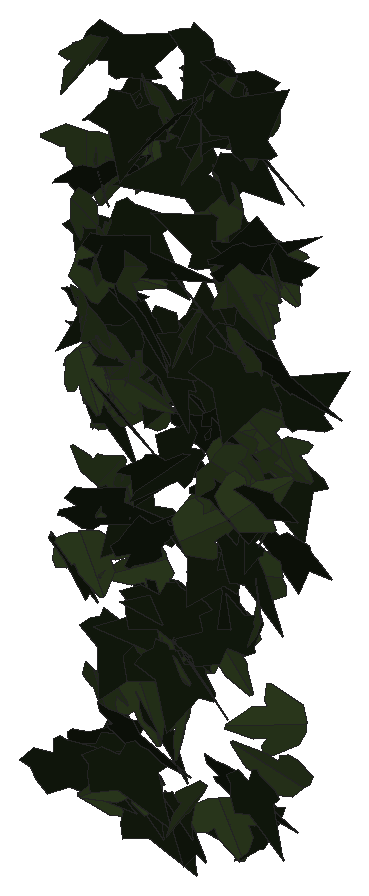
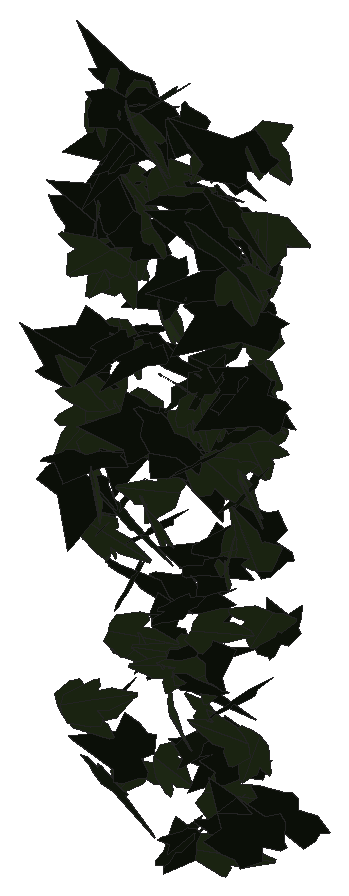
# SketchUp Ruby script. Lengths in inches.
U = 1.inch
M = Sketchup.active_model
def pt(a) = Geom::Point3d.new(a.map { |v| v * U })
def face(e, loops, mat)
  f = e.add_face(loops[0].map { |a| pt(a) })
  loops[1..].each { |l| e.add_face(l.map { |a| pt(a) }).erase! }
  f.material = f.back_material = mat if mat
  f
end
# faces: each face lists its corners as indices into pts; further lists are holes
def faces(e, pts, list, mat = nil) = list.each { |f| face(e, (f[0].is_a?(Array) ? f : [f]).map { |l| l.map { |i| pts[i] } }, mat) }
# xy, xz, yz: faces in a plane at the given z, y or x. An outline is a flat list of corners, or four numbers for a rectangle; further outlines are holes
def ring(l) = l.size == 4 ? [[l[0], l[1]], [l[2], l[1]], [l[2], l[3]], [l[0], l[3]]] : l.each_slice(2).to_a
def flat(e, list, mat, &to3) = list.each { |f| face(e, (f[0].is_a?(Array) ? f : [f]).map { |l| ring(l).map { |u, v| to3.(u, v) } }, mat) }
def xy(e, z, list, mat = nil) = flat(e, list, mat) { |x, y| [x, y, z] }
def xz(e, y, list, mat = nil) = flat(e, list, mat) { |x, z| [x, y, z] }
def yz(e, x, list, mat = nil) = flat(e, list, mat) { |y, z| [x, y, z] }
def lines(e, pts, list) = list.each { |a, b| e.add_line(pt(pts[a]), pt(pts[b])) }
# prism: a flat outline (further loops are holes) pulled along v
def prism(e, loops, v, mat = nil)
  f = face(e, loops, mat); d = Geom::Vector3d.new(v.map { |x| x * U })
  f.pushpull(f.normal.samedirection?(d) ? d.length : -d.length)
end
def box(e, o, s, mat = nil) = prism(e, [[o, [o[0] + s[0], o[1], o[2]], [o[0] + s[0], o[1] + s[1], o[2]], [o[0], o[1] + s[1], o[2]]]], [0, 0, s[2]], mat)
def at(x, y, z, deg = 0) = Geom::Transformation.translation(pt([x, y, z])) * Geom::Transformation.rotation(ORIGIN, Z_AXIS, deg.degrees)
def axes(o, x, y, z) = Geom::Transformation.new([*x, 0, *y, 0, *z, 0, *pt(o).to_a, 1])
def part(name) = M.definitions.add(name)
# library, detail: a bought-in or finely detailed component or shape, given as its bounding box
def library(name, o, s) = part(name).tap { |d| box(d.entities, o, s) }
def detail(e, o, s) = box(e.add_group.entities, o, s)
def put(e, d, t, mat = nil) = e.add_instance(d, t).tap { |i| i.material = mat if mat }
def group(e, t, mat = nil) = e.add_group.tap { |g| g.transformation = t; g.material = mat if mat }.entities
root = M.entities
M.materials.add("1026 AP 7946 SUNNY SIDE UP").color = [254, 231, 186]
M.materials.add("efeu1").color = [18, 25, 13]
M.materials.add("efeu2").color = [43, 57, 29]
c1 = part("ivyleaf_10")
p = [[0,0.5,-0.03],[-0.0625,2.02,-0.43],[-0.19,2.01,-0.46],[-0.54,1.05,-0.29],[-0.52,0.625,-0.18],[-0.83,0.76,-0.28],
  [-1.16,0.64,-0.33],[-1.15,0.33,-0.24],[-0.77,-0.39,0.02],[-0.3,-0.51,0.16],[0.04,-0.48,0.23],[-0.02,2.01,-0.4375],
  [-0.06,2.01,-0.43],[0.04,-0.49,0.23],[0.67,-0.49,0.14],[1.38,0.36,-0.2],[1.375,0.51,-0.24],[0.81,0.65,-0.19],
  [0.62,0.59,-0.15],[0.6,1.09,-0.28],[0.5,1.23,-0.31]]
faces(c1.entities,p,[[0,1,2,3,4,5,6,7,8,9,10],[11,12,0,13,14,15,16,17,18,19,20]],"efeu2")
c2 = part("ivyleaf_9")
p = [[1.54,2.16,1.25],[1.36,2.04,1.19],[-0.21,0.99,0.68],[-0.71,1.11,0.82],[-0.85,0.86,0.67],[-0.8,0.17,0.21],
  [-0.9,-0.01,0.1],[-0.67,-0.16,-0.02],[-0.08,-0.08,-0.05],[-0.03,-0.6,-0.4],[0.65,-0.88,-0.66],[0.83,-0.6,-0.49],
  [1.29,-0.42,-0.43],[1.8125,-0.07,-0.26],[1.21,0.44,0.15]]
faces(c2.entities,p,[[0,1,2,3,4,5,6,7,8,9,10,11,12,13,14]],"efeu1")
put(root,c1,axes([125.12,211.6,276.24],[-0.30971,0.08438,0.28266],[0.40804,-0.08857,0.21984],[0.1913,0.32553,-0.01128]),"1026 AP 7946 SUNNY SIDE UP")
put(root,c2,axes([126.02,211.5,273.74],[0.08468,0.26535,-0.18565],[-0.0411,-0.18002,-0.27985],[-0.50402,0.05926,-0.00837]),"1026 AP 7946 SUNNY SIDE UP")
put(root,c2,axes([126.16,211.55,278.82],[-0.20277,0.23701,-0.16333],[0.09037,-0.15033,-0.2782],[-0.44036,-0.13998,0.01811]),"1026 AP 7946 SUNNY SIDE UP")
put(root,c1,axes([127,211.62,276.72],[-0.33741,0.11008,-0.27658],[0.31923,-0.18267,-0.24483],[-0.32724,-0.2917,0.04633]),"1026 AP 7946 SUNNY SIDE UP")
put(root,c2,axes([127.09,211.51,278.92],[-0.22211,0.14991,0.2901],[0.32473,-0.19053,0.21075],[0.38078,0.24994,-0.01051]),"1026 AP 7946 SUNNY SIDE UP")
put(root,c2,axes([125.28,211.53,269.14],[-0.03055,-0.2161,-0.22105],[0.11388,0.20432,-0.21881],[0.46372,-0.06441,0.03917]),"1026 AP 7946 SUNNY SIDE UP")
put(root,c1,axes([126.95,211.41,274.0625],[-0.13765,-0.21772,-0.24],[0.20403,0.19497,-0.23807],[0.45645,-0.15281,0.03404]),"1026 AP 7946 SUNNY SIDE UP")
put(root,c2,axes([124.92,211.61,274.3],[0.3457,-0.17847,0.06715],[0.05909,-0.05845,-0.29125],[0.29342,0.22204,-0.02047]),"1026 AP 7946 SUNNY SIDE UP")
put(root,c1,axes([126.33,211.6875,275.83],[0.15419,-0.27095,0.12188],[0.04264,-0.1175,-0.29722],[0.46391,0.10086,-0.01319]),"1026 AP 7946 SUNNY SIDE UP")
put(root,c2,axes([127.31,211.62,269.43],[0.16228,-0.2843,-0.07382],[-0.06451,0.05949,-0.3107],[0.45586,0.10963,-0.01769]),"1026 AP 7946 SUNNY SIDE UP")
put(root,c2,axes([127.18,211.46,273.73],[0.42834,0.15969,-0.14948],[-0.17686,-0.09604,-0.32496],[-0.29066,0.29378,-0.02257]),"1026 AP 7946 SUNNY SIDE UP")
put(root,c2,axes([125.08,211.39,276.48],[0.39253,0.08741,0.26918],[0.40942,0.0384,-0.2698],[-0.13938,0.35897,-0.03444]),"1026 AP 7946 SUNNY SIDE UP")
put(root,c1,axes([125.26,211.59,274.625],[0.03815,-0.00602,0.29977],[0.45738,0.01135,-0.02468],[-0.01701,0.29181,0.00886]),"1026 AP 7946 SUNNY SIDE UP")
put(root,c2,axes([124.73,211.4,272.69],[0.34005,0.10747,0.23171],[0.34174,0.06289,-0.24654],[-0.19017,0.30517,-0.02871]),"1026 AP 7946 SUNNY SIDE UP")
put(root,c2,axes([127.09,211.78,275.27],[-0.23418,-0.2826,0.02912],[-0.00061,-0.03352,-0.32891],[0.44683,-0.14815,0.01481]),"1026 AP 7946 SUNNY SIDE UP")
put(root,c2,axes([124.88,211.5,277.64],[0.11895,0.28671,-0.08881],[-0.0333,-0.08525,-0.30597],[-0.47032,0.07855,-0.0008]),"1026 AP 7946 SUNNY SIDE UP")
put(root,c1,axes([125.05,211.35,276.43],[0.10038,-0.0414,0.37634],[-0.32327,0.30365,0.07419],[-0.47969,-0.2133,0.02875]),"1026 AP 7946 SUNNY SIDE UP")
put(root,c2,axes([124.24,211.83,271.49],[-0.00484,-0.17117,0.26038],[0.10676,-0.24779,-0.17282],[0.46926,0.05461,0.042]),"1026 AP 7946 SUNNY SIDE UP")
put(root,c1,axes([126.29,211.79,268.85],[0.06161,-0.21932,0.21022],[0.03119,-0.2047,-0.23038],[0.47135,0.04221,-0.01223]),"1026 AP 7946 SUNNY SIDE UP")
put(root,c2,axes([126.1875,211.66,276.29],[0.39564,-0.19646,0.02072],[0.00176,-0.03295,-0.32803],[0.3107,0.25035,-0.02452]),"1026 AP 7946 SUNNY SIDE UP")
put(root,c2,axes([126.23,211.7,273.91],[-0.46209,0.13322,-0.12073],[0.14856,-0.07614,-0.33155],[-0.23707,-0.30737,0.02755]),"1026 AP 7946 SUNNY SIDE UP")
put(root,c2,axes([125.85,211.63,271.64],[-0.14687,-0.12827,-0.27634],[0.31991,0.17642,-0.1593],[0.33952,-0.22173,0.03056]),"1026 AP 7946 SUNNY SIDE UP")
put(root,c2,axes([126.53,211.87,272.42],[-0.1496,-0.25042,0.15774],[-0.05748,-0.1511,-0.27631],[0.45912,-0.10051,0.01681]),"1026 AP 7946 SUNNY SIDE UP")
put(root,c2,axes([125.33,211.76,278.52],[-0.37869,-0.07665,-0.18426],[0.29452,-0.01666,-0.25318],[0.08059,-0.29927,0.05941]),"1026 AP 7946 SUNNY SIDE UP")
put(root,c1,axes([126.55,211.49,278.5625],[0.06983,-0.26487,-0.2432],[-0.03165,0.23414,-0.27492],[0.55542,0.04664,0.01491]),"1026 AP 7946 SUNNY SIDE UP")
put(root,c1,axes([127.29,211.43,273.54],[0.19729,0.10733,-0.30542],[0.30849,0.22405,0.17006],[0.38926,-0.23195,0.02003]),"1026 AP 7946 SUNNY SIDE UP")
put(root,c1,axes([125.33,211.84,268.78],[0.15458,0.07911,-0.33089],[-0.33001,-0.24469,-0.12951],[-0.40293,0.23075,-0.02087]),"1026 AP 7946 SUNNY SIDE UP")
put(root,c2,axes([124.18,211.59,268.77],[0.0055,-0.05249,-0.31572],[0.32346,0.22983,-0.03683],[0.366,-0.20232,0.03729]),"1026 AP 7946 SUNNY SIDE UP")
put(root,c1,axes([124.83,211.64,275.13],[-0.43077,0.1254,-0.02626],[0.02055,-0.03418,-0.30947],[-0.20038,-0.27308,0.02472]),"1026 AP 7946 SUNNY SIDE UP")
put(root,c1,axes([124.71,211.6,275.43],[-0.36428,0.14915,0.1485],[-0.21635,0.04953,-0.28197],[-0.24283,-0.26787,0.02844]),"1026 AP 7946 SUNNY SIDE UP")
put(root,c2,axes([126.23,211.65,270.92],[0.39463,-0.13734,-0.10286],[-0.15431,0.02637,-0.29365],[0.21699,0.26852,-0.02177]),"1026 AP 7946 SUNNY SIDE UP")
put(root,c1,axes([124.56,211.84,279.16],[-0.00909,-0.30607,0.16579],[-0.01714,-0.16245,-0.31624],[0.54475,-0.01022,-0.00718]),"1026 AP 7946 SUNNY SIDE UP")
put(root,c2,axes([126.375,211.85,277.93],[-0.39497,-0.05239,0.1896],[-0.2686,-0.07657,-0.26265],[0.13661,-0.30202,0.03176]),"1026 AP 7946 SUNNY SIDE UP")
put(root,c1,axes([126.47,211.47,272.87],[0.10422,0.06933,-0.33181],[0.3061,0.2573,0.09971],[0.41868,-0.20537,0.0097]),"1026 AP 7946 SUNNY SIDE UP")
put(root,c2,axes([127.05,211.5,277],[0.18894,0.28554,-0.15961],[0.04138,0.15781,0.31826],[0.51037,-0.1185,0.03329]),"1026 AP 7946 SUNNY SIDE UP")
put(root,c1,axes([127.53,211.49,272.04],[0.01747,-0.10018,-0.32543],[-0.11646,0.30674,-0.10129],[0.50703,0.07391,-0.01205]),"1026 AP 7946 SUNNY SIDE UP")
put(root,c2,axes([125.98,211.9,270.5625],[-0.15623,-0.28157,0.05652],[-0.01499,-0.05648,-0.30777],[0.4513,-0.09935,0.00934]),"1026 AP 7946 SUNNY SIDE UP")
put(root,c2,axes([126.95,211.57,271.37],[-0.5334,0.05893,-0.07586],[-0.10529,0.04487,0.35342],[0.10502,0.34428,-0.03097]),"1026 AP 7946 SUNNY SIDE UP")
put(root,c2,axes([126.11,211.94,271.36],[-0.02787,-0.23721,-0.17152],[-0.00943,-0.16512,0.24403],[-0.45438,0.01798,0.00545]),"1026 AP 7946 SUNNY SIDE UP")
put(root,c2,axes([124.99,211.8,269.39],[0.30628,-0.12715,0.19905],[0.23938,-0.12094,-0.23992],[0.27507,0.24683,-0.01285]),"1026 AP 7946 SUNNY SIDE UP")
put(root,c2,axes([125.71,211.91,274.97],[0.10579,-0.29897,0.09703],[0.02124,-0.09521,-0.31616],[0.49322,0.06822,-0.00719]),"1026 AP 7946 SUNNY SIDE UP")
put(root,c1,axes([124.56,211.57,276.96],[-0.03276,0.22476,0.2126],[-0.11722,0.19554,-0.22742],[-0.46386,-0.06528,0.04246]),"1026 AP 7946 SUNNY SIDE UP")
put(root,c1,axes([125.46,211.78,274.89],[-0.10867,-0.29571,0.00388],[0.00849,-0.00685,-0.31281],[0.46497,-0.06899,0.00662]),"1026 AP 7946 SUNNY SIDE UP")
put(root,c2,axes([126.99,211.8125,272.66],[0.2428,-0.30885,-0.07115],[-0.07113,0.05255,-0.355],[0.49192,0.16004,-0.01621]),"1026 AP 7946 SUNNY SIDE UP")
put(root,c1,axes([124.55,211.76,277.84],[-0.46187,-0.12098,0.01335],[-0.00274,-0.03146,-0.32614],[0.19141,-0.29236,0.02754]),"1026 AP 7946 SUNNY SIDE UP")
put(root,c1,axes([124.51,211.74,274.56],[0.1315,0.30795,0.0233],[0.02393,0.01748,-0.32847],[-0.48474,0.0844,-0.0099]),"1026 AP 7946 SUNNY SIDE UP")
put(root,c2,axes([127.28,211.87,276.9],[0.47735,0.00253,0.1519],[-0.23101,0.03397,0.31125],[-0.01978,-0.33577,0.03065]),"1026 AP 7946 SUNNY SIDE UP")
put(root,c1,axes([124.69,211.68,276.09],[-0.06942,-0.11133,-0.33527],[0.48278,0.13381,-0.08946],[0.24171,-0.29924,0.08239]),"1026 AP 7946 SUNNY SIDE UP")
put(root,c2,axes([125.1,211.98,275.59],[0.18015,-0.2747,0.13745],[0.06407,-0.12916,-0.30716],[0.47698,0.1211,-0.01066]),"1026 AP 7946 SUNNY SIDE UP")
put(root,c2,axes([126.63,212,276.92],[-0.02157,0.01555,0.33982],[-0.45155,-0.16338,-0.00533],[0.25607,-0.28678,0.01923]),"1026 AP 7946 SUNNY SIDE UP")
put(root,c1,axes([125.3,211.9,269.94],[0.38624,-0.03306,0.17173],[0.25787,-0.03194,-0.25538],[0.07114,0.29524,-0.00663]),"1026 AP 7946 SUNNY SIDE UP")
put(root,c2,axes([125.28,211.75,275.03],[-0.18256,0.22853,0.14656],[-0.27483,0.05227,-0.23528],[-0.32051,-0.17499,0.11827]),"1026 AP 7946 SUNNY SIDE UP")
put(root,c1,axes([124.99,212.06,272.77],[0.0483,0.09115,-0.30154],[-0.12631,-0.28204,-0.10064],[-0.46601,0.08589,-0.00398]),"1026 AP 7946 SUNNY SIDE UP")
put(root,c1,axes([126.68,211.85,268.72],[0.38508,0.12617,0.11118],[0.1634,0.03187,-0.28302],[-0.20267,0.26543,-0.01694]),"1026 AP 7946 SUNNY SIDE UP")
put(root,c2,axes([125.375,211.65,272.15],[0.06679,-0.00556,0.34623],[0.39261,0.22735,-0.0273],[-0.3539,0.25117,0.03505]),"1026 AP 7946 SUNNY SIDE UP")
put(root,c2,axes([124.86,212.12,270.44],[-0.13108,-0.27149,0.16816],[-0.06039,-0.16048,-0.29336],[0.49569,-0.09134,0.00873]),"1026 AP 7946 SUNNY SIDE UP")
put(root,c1,axes([124.41,211.85,271.8125],[0.36612,0.1756,0.09049],[0.12815,0.03582,-0.29955],[-0.28011,0.24591,-0.01877]),"1026 AP 7946 SUNNY SIDE UP")
put(root,c1,axes([125.39,211.98,270.63],[-0.1457,0.03591,-0.28214],[0.34908,-0.16254,-0.10021],[-0.25894,-0.23933,0.02365]),"1026 AP 7946 SUNNY SIDE UP")
put(root,c1,axes([126.68,211.96,273.96],[0.24528,0.00714,0.30384],[0.4603,-0.04481,-0.15867],[0.0571,0.33059,-0.0261]),"1026 AP 7946 SUNNY SIDE UP")
put(root,c2,axes([126.74,212.11,278.99],[-0.36396,-0.18738,0.11619],[-0.10581,-0.09685,-0.30572],[0.32812,-0.23908,0.03029]),"1026 AP 7946 SUNNY SIDE UP")
put(root,c1,axes([126.89,211.74,277.71],[0.08368,-0.10789,-0.34553],[-0.34892,0.25242,-0.11867],[0.42914,0.22628,-0.0291]),"1026 AP 7946 SUNNY SIDE UP")
put(root,c1,axes([126.61,212.04,279.19],[0.07574,-0.28277,0.14079],[0.0668,-0.13276,-0.29572],[0.49041,0.06176,0.01854]),"1026 AP 7946 SUNNY SIDE UP")
put(root,c1,axes([124.74,211.75,277.49],[-0.20657,0.24117,0.20491],[-0.21183,0.14939,-0.27932],[-0.44205,-0.18429,0.03809]),"1026 AP 7946 SUNNY SIDE UP")
put(root,c1,axes([125.86,212.08,269.82],[0.25485,-0.15816,0.21165],[0.19425,-0.16711,-0.23289],[0.35971,0.2023,-0.02419]),"1026 AP 7946 SUNNY SIDE UP")
put(root,c1,axes([125.48,211.92,278.77],[-0.34263,0.21182,-0.06327],[0.04493,-0.06018,-0.31254],[-0.3444,-0.21858,0.02216]),"1026 AP 7946 SUNNY SIDE UP")
put(root,c1,axes([127.24,211.96,278.86],[-0.08256,-0.3331,-0.00514],[0.00825,0.00231,-0.34735],[0.52373,-0.05255,0.00466]),"1026 AP 7946 SUNNY SIDE UP")
put(root,c2,axes([125.41,212.07,269.59],[0.17312,-0.26039,0.09531],[0.0362,-0.09219,-0.29143],[0.43379,0.11161,-0.01372]),"1026 AP 7946 SUNNY SIDE UP")
put(root,c1,axes([127.09,211.85,276.55],[-0.27011,-0.23773,-0.1611],[0.18533,0.10509,-0.29995],[0.40596,-0.20615,0.02974]),"1026 AP 7946 SUNNY SIDE UP")
put(root,c2,axes([127.08,211.95,272.73],[-0.40316,0.185,-0.02542],[0.00592,-0.03856,-0.32457],[-0.29363,-0.25478,0.02835]),"1026 AP 7946 SUNNY SIDE UP")
put(root,c1,axes([125.49,212.17,277.72],[-0.00555,-0.09921,0.30729],[0.10586,-0.29219,-0.10082],[0.48367,0.06281,0.02559]),"1026 AP 7946 SUNNY SIDE UP")
put(root,c1,axes([127.42,211.9,277.07],[-0.24087,0.25751,0.01716],[-0.04079,0.0022,-0.30789],[-0.40355,-0.15392,0.02088]),"1026 AP 7946 SUNNY SIDE UP")
put(root,c2,axes([125.69,212.14,270.83],[-0.21655,-0.04264,0.26999],[-0.34361,-0.14997,-0.14418],[0.23782,-0.25551,0.03753]),"1026 AP 7946 SUNNY SIDE UP")
put(root,c1,axes([124.57,211.99,272.76],[-0.41133,0.05628,0.1514],[0.23645,0.00744,0.27346],[0.07136,0.2998,-0.03339]),"1026 AP 7946 SUNNY SIDE UP")
put(root,c2,axes([126.625,212.22,271.58],[-0.03936,-0.13138,0.28394],[-0.07585,-0.27213,-0.13936],[0.47515,-0.05432,0.00127]),"1026 AP 7946 SUNNY SIDE UP")
put(root,c1,axes([126.91,212.03,276.41],[-0.3814,0.07553,-0.18106],[0.21537,-0.13049,-0.25267],[-0.21087,-0.2699,0.06942]),"1026 AP 7946 SUNNY SIDE UP")
put(root,c2,axes([124.68,212.15,275.32],[-0.02125,0.06408,-0.3073],[0.06272,-0.29602,-0.06902],[-0.47619,-0.04185,0.00462]),"1026 AP 7946 SUNNY SIDE UP")
put(root,c2,axes([126.43,211.85,275.16],[-0.52512,0.0516,0.06468],[0.10409,0.02079,0.34686],[0.07352,0.33912,-0.02907]),"1026 AP 7946 SUNNY SIDE UP")
put(root,c2,axes([124.5,212.03,273.99],[0.24125,-0.26374,-0.06393],[-0.07106,0.04367,-0.3136],[0.41953,0.15906,-0.01635]),"1026 AP 7946 SUNNY SIDE UP")
put(root,c1,axes([124.58,211.98,269.83],[-0.40173,0.15505,-0.03318],[0.02339,-0.03904,-0.30698],[-0.24819,-0.25465,0.02479]),"1026 AP 7946 SUNNY SIDE UP")
put(root,c2,axes([125.23,212.2,272.5],[-0.31767,-0.20844,0.09401],[-0.0808,-0.07871,-0.29899],[0.34932,-0.20776,0.01634]),"1026 AP 7946 SUNNY SIDE UP")
put(root,c1,axes([124.54,212.06,274.49],[0.36699,0.15946,-0.07638],[-0.06757,-0.0693,-0.28975],[-0.26875,0.23517,-0.03146]),"1026 AP 7946 SUNNY SIDE UP")
put(root,c1,axes([127.28,212.05,272.28],[-0.13478,0.04351,0.29092],[-0.43504,-0.08529,-0.07354],[0.11067,-0.28228,0.06522]),"1026 AP 7946 SUNNY SIDE UP")
put(root,c1,axes([126.24,212.14,277.37],[0.28063,-0.10035,0.23722],[0.3287,-0.09854,-0.2112],[0.22047,0.27464,0.01293]),"1026 AP 7946 SUNNY SIDE UP")
put(root,c1,axes([127.22,211.78,278.98],[-0.05,0.02787,-0.3705],[-0.20161,0.33675,0.04051],[0.53042,0.13063,-0.01953]),"1026 AP 7946 SUNNY SIDE UP")
put(root,c2,axes([126.5,212.1,269.02],[0.30513,-0.13458,0.2057],[0.23957,-0.13121,-0.24349],[0.29447,0.2462,-0.01504]),"1026 AP 7946 SUNNY SIDE UP")
put(root,c1,axes([126.89,211.99,275.48],[-0.35293,0.11103,0.15741],[-0.25645,0.00388,-0.25073],[-0.1482,-0.27114,0.05902]),"1026 AP 7946 SUNNY SIDE UP")
put(root,c2,axes([125.22,212.26,275.23],[0.04002,-0.20284,0.23785],[0.08791,-0.22592,-0.2111],[0.47656,0.05871,0.01897]),"1026 AP 7946 SUNNY SIDE UP")
put(root,c1,axes([127.56,212.1,269.38],[-0.25587,-0.02251,-0.27196],[-0.41222,-0.03013,0.16903],[-0.05892,0.30854,-0.00151]),"1026 AP 7946 SUNNY SIDE UP")
put(root,c2,axes([125.02,212.13,268.67],[0.12662,-0.28212,-0.03195],[-0.02546,0.02595,-0.30197],[0.44528,0.08171,-0.00818]),"1026 AP 7946 SUNNY SIDE UP")
put(root,c2,axes([126.15,212.3125,279.36],[-0.1726,-0.22264,0.20578],[-0.03677,-0.20705,-0.25061],[0.47023,-0.09791,0.05594]),"1026 AP 7946 SUNNY SIDE UP")
put(root,c2,axes([125.66,212.17,270.54],[-0.46651,-0.01409,0.06283],[-0.09259,-0.03856,-0.30408],[0.03375,-0.30044,0.03429]),"1026 AP 7946 SUNNY SIDE UP")
put(root,c2,axes([126.74,212.11,278.59],[0.40627,-0.19772,0.06359],[0.05361,-0.05855,-0.3345],[0.32179,0.25938,-0.02456]),"1026 AP 7946 SUNNY SIDE UP")
put(root,c2,axes([127.51,211.99,272.94],[0.45095,0.03055,-0.18007],[-0.26633,-0.05298,-0.29585],[-0.08407,0.33174,-0.02866]),"1026 AP 7946 SUNNY SIDE UP")
put(root,c1,axes([124.81,212.26,272.61],[-0.01772,-0.02789,0.30191],[0.29766,-0.22549,-0.01592],[0.35481,0.18777,0.02843]),"1026 AP 7946 SUNNY SIDE UP")
put(root,c1,axes([125.16,212.17,274.03],[-0.32521,-0.11348,0.2351],[-0.26966,-0.15655,-0.24055],[0.29768,-0.26579,0.03893]),"1026 AP 7946 SUNNY SIDE UP")
put(root,c1,axes([125.56,212.08,278.12],[0.31973,0.23241,0.00829],[0.02793,-0.00662,-0.31765],[-0.36453,0.20334,-0.01707]),"1026 AP 7946 SUNNY SIDE UP")
put(root,c1,axes([125.98,212.18,278.28],[-0.0992,-0.29413,0.0988],[-0.01302,-0.09794,-0.31023],[0.4871,-0.06252,0.01183]),"1026 AP 7946 SUNNY SIDE UP")
put(root,c2,axes([126.33,211.89,278.73],[0.03988,-0.06076,-0.33205],[-0.03239,0.322,-0.06239],[0.51419,0.02499,0.02182]),"1026 AP 7946 SUNNY SIDE UP")
put(root,c2,axes([125.65,212.33,267.97],[-0.01808,-0.20229,0.23519],[0.03603,-0.22953,-0.20863],[0.47962,0.00961,0.02454]),"1026 AP 7946 SUNNY SIDE UP")
put(root,c2,axes([126.8,211.96,278.3],[0.14558,-0.14739,-0.29556],[-0.19969,0.25677,-0.17713],[0.46493,0.15644,0.01647]),"1026 AP 7946 SUNNY SIDE UP")
put(root,c1,axes([126.1875,212.2,272.93],[0.35174,-0.1956,0.07289],[0.06157,-0.0641,-0.30567],[0.32183,0.22604,-0.02119]),"1026 AP 7946 SUNNY SIDE UP")
put(root,c2,axes([125.79,212.16,274.125],[0.23089,0.00327,-0.30557],[0.45682,0.06535,0.14928],[0.09433,-0.32447,0.02501]),"1026 AP 7946 SUNNY SIDE UP")
put(root,c1,axes([125.11,212.22,268.1],[0.05647,-0.02806,-0.30672],[-0.44761,-0.09456,-0.02676],[-0.14324,0.28442,-0.03729]),"1026 AP 7946 SUNNY SIDE UP")
put(root,c2,axes([127.1875,212.03,268.51],[-0.27602,0.2432,0.08352],[-0.10288,0.05077,-0.30782],[-0.38904,-0.18598,0.02215]),"1026 AP 7946 SUNNY SIDE UP")
put(root,c1,axes([124.75,212.21,269.96],[-0.11846,-0.00713,-0.29876],[0.39858,-0.14723,-0.06498],[-0.22167,-0.26092,0.04282]),"1026 AP 7946 SUNNY SIDE UP")
put(root,c2,axes([125.5625,212.3,275.19],[-0.4054,-0.08739,-0.10668],[0.20158,-0.08808,-0.25398],[0.06711,-0.26332,0.11848]),"1026 AP 7946 SUNNY SIDE UP")
put(root,c2,axes([127.07,212.21,275.21],[0.32564,-0.13479,0.20337],[0.24621,-0.12219,-0.25491],[0.2853,0.25929,-0.01214]),"1026 AP 7946 SUNNY SIDE UP")
put(root,c2,axes([125.36,212.14,268.18],[-0.06417,-0.21051,-0.20962],[0.0881,0.19481,-0.21936],[0.45053,-0.06808,0.01304]),"1026 AP 7946 SUNNY SIDE UP")
put(root,c1,axes([125.33,212.2,274.96],[-0.23121,-0.26729,0.01969],[-0.00154,-0.023,-0.31424],[0.42154,-0.14669,0.00965]),"1026 AP 7946 SUNNY SIDE UP")
put(root,c2,axes([124.7,212.09,276.54],[-0.04489,-0.18277,-0.34642],[0.17848,0.3169,-0.1861],[0.57322,-0.11298,0.03081]),"1026 AP 7946 SUNNY SIDE UP")
put(root,c1,axes([125.16,212.36,271.59],[0.12365,0.04083,-0.29598],[-0.31027,-0.21107,-0.0877],[-0.33507,0.21051,-0.02802]),"1026 AP 7946 SUNNY SIDE UP")
put(root,c1,axes([127.03,212.34,273.97],[0.17234,0.09933,-0.25621],[-0.2625,-0.18555,-0.15288],[-0.33031,0.19928,-0.01218]),"1026 AP 7946 SUNNY SIDE UP")
put(root,c1,axes([124.48,212.27,273.98],[0.28386,-0.23158,0.03655],[0.01203,-0.04059,-0.30211],[0.3685,0.17971,-0.01829]),"1026 AP 7946 SUNNY SIDE UP")
put(root,c1,axes([126.26,212.27,270.85],[0.28605,-0.00312,0.27121],[0.40657,-0.05828,-0.18511],[0.07813,0.31467,-0.02969]),"1026 AP 7946 SUNNY SIDE UP")
put(root,c1,axes([127.3,212.1,273.23],[0.11304,-0.26398,-0.20799],[-0.09653,0.1909,-0.28064],[0.51211,0.09425,-0.00699]),"1026 AP 7946 SUNNY SIDE UP")
put(root,c1,axes([126.81,212.22,274.27],[0.28684,0.01178,0.25853],[0.39183,0.03022,-0.18795],[-0.0493,0.30872,0.01036]),"1026 AP 7946 SUNNY SIDE UP")
put(root,c2,axes([126.57,212.23,279.28],[0.2022,0.14823,-0.26899],[-0.21101,-0.22674,-0.20137],[-0.42362,0.18369,-0.02809]),"1026 AP 7946 SUNNY SIDE UP")
put(root,c2,axes([124.34,212.08,275.4],[0.45876,0.10543,0.08358],[0.1333,0.0015,-0.31841],[-0.16046,0.30266,-0.02555]),"1026 AP 7946 SUNNY SIDE UP")
put(root,c2,axes([124.64,212.14,278.875],[-0.04221,-0.02023,0.328],[0.50171,0.00487,0.02805],[-0.01031,0.31959,0.02221]),"1026 AP 7946 SUNNY SIDE UP")
put(root,c1,axes([125.49,212.07,270.91],[0.07368,0.0072,-0.33509],[0.43874,0.16821,0.04622],[0.26323,-0.28237,0.01675]),"1026 AP 7946 SUNNY SIDE UP")
put(root,c2,axes([125.05,212.04,277.62],[0.09142,0.27895,-0.15752],[0.03855,0.15266,0.29436],[0.49991,-0.06278,0.00611]),"1026 AP 7946 SUNNY SIDE UP")
put(root,c2,axes([124.8125,212.16,268.51],[-0.39098,-0.08264,0.14458],[0.19877,0.06493,0.2696],[-0.16249,0.27828,-0.01811]),"1026 AP 7946 SUNNY SIDE UP")
put(root,c2,axes([126.26,212.49,274.42],[-0.29236,-0.12332,0.18699],[-0.10454,-0.19591,-0.20764],[0.32978,-0.17143,0.09995]),"1026 AP 7946 SUNNY SIDE UP")
put(root,c1,axes([127.3,212.17,274.03],[-0.24415,-0.18836,-0.18644],[0.20502,0.1251,-0.25014],[0.35455,-0.20205,0.01626]),"1026 AP 7946 SUNNY SIDE UP")
put(root,c1,axes([124.5625,212.34,277.23],[-0.22978,-0.26172,0.079],[-0.02266,-0.08114,-0.30811],[0.4289,-0.14451,0.02604]),"1026 AP 7946 SUNNY SIDE UP")
put(root,c1,axes([126.43,212.23,278.95],[0.3302,-0.15387,-0.20517],[-0.25126,0.1174,-0.26751],[0.30433,0.26388,0.00175]),"1026 AP 7946 SUNNY SIDE UP")
put(root,c1,axes([125.61,212.23,274.6],[-0.34839,0.14893,0.11286],[-0.19783,0.00212,-0.26715],[-0.21194,-0.24679,0.06384]),"1026 AP 7946 SUNNY SIDE UP")
put(root,c1,axes([125.73,212.09,270.72],[0.06259,-0.00925,-0.31243],[0.32726,0.22333,0.02244],[0.34704,-0.20893,0.03519]),"1026 AP 7946 SUNNY SIDE UP")
put(root,c1,axes([126.53,212.41,271.1],[0.09565,0.04704,-0.28607],[-0.37694,-0.141,-0.07945],[-0.23325,0.24714,0.01109]),"1026 AP 7946 SUNNY SIDE UP")
put(root,c1,axes([126.96,212.27,276.78],[0.35722,0.11508,0.19275],[0.27028,0.07293,-0.26172],[-0.21363,0.2847,-0.00883]),"1026 AP 7946 SUNNY SIDE UP")
put(root,c2,axes([127.34,212.27,274.67],[-0.17853,0.0801,0.28989],[0.41392,-0.10266,0.13915],[0.19921,0.2851,-0.02933]),"1026 AP 7946 SUNNY SIDE UP")
put(root,c2,axes([125.2,212.22,271],[0.03573,-0.08133,0.2977],[-0.13181,0.27703,0.0886],[-0.45399,-0.08683,-0.0023]),"1026 AP 7946 SUNNY SIDE UP")
put(root,c2,axes([126.14,212.28,275.5625],[0.09694,-0.20743,-0.22785],[-0.0229,0.22223,-0.21876],[0.47489,0.05306,0.03596]),"1026 AP 7946 SUNNY SIDE UP")
put(root,c2,axes([126.36,212.125,274.14],[0.1327,0.05855,0.29792],[0.34158,0.1907,-0.10409],[-0.3132,0.23279,0.0127]),"1026 AP 7946 SUNNY SIDE UP")
put(root,c2,axes([126.59,212.25,275.57],[0.1067,-0.18463,-0.25512],[-0.06815,0.24427,-0.19927],[0.47956,0.07579,0.02844]),"1026 AP 7946 SUNNY SIDE UP")
put(root,c2,axes([125.11,212.22,277.625],[-0.17651,0.27722,0.09503],[-0.15773,0.05453,-0.29939],[-0.43065,-0.1336,0.07071]),"1026 AP 7946 SUNNY SIDE UP")
put(root,c2,axes([125.65,212.41,274.5],[-0.18071,-0.07514,-0.29627],[0.43548,0.08364,-0.13624],[0.16792,-0.29778,0.0345]),"1026 AP 7946 SUNNY SIDE UP")
put(root,c1,axes([127.02,212.3,274.53],[-0.33997,-0.1318,0.18763],[0.21799,0.12207,0.2602],[-0.2795,0.25552,-0.02529]),"1026 AP 7946 SUNNY SIDE UP")
put(root,c2,axes([124.2,212.33,268.5625],[0.40294,0.17668,0.00717],[-0.04327,0.02951,0.31818],[0.27457,-0.25462,0.03962]),"1026 AP 7946 SUNNY SIDE UP")
put(root,c2,axes([125.13,212.57,274.28],[-0.13062,-0.25228,0.12013],[-0.01935,-0.11974,-0.27325],[0.43753,-0.08061,0.02378]),"1026 AP 7946 SUNNY SIDE UP")
put(root,c2,axes([125.38,212.51,278.32],[-0.2243,-0.27067,-0.0465],[0.08048,0.02199,-0.31303],[0.4235,-0.14753,0.03486]),"1026 AP 7946 SUNNY SIDE UP")
put(root,c2,axes([124.89,212.33,278.38],[-0.30836,0.24432,-0.03707],[0.01601,-0.03968,-0.32252],[-0.38831,-0.19565,0.01614]),"1026 AP 7946 SUNNY SIDE UP")
put(root,c2,axes([127.14,212.44,273.64],[-0.13275,-0.26459,-0.14113],[0.12165,0.11644,-0.28323],[0.45132,-0.10921,0.03483]),"1026 AP 7946 SUNNY SIDE UP")
put(root,c1,axes([127.14,212.6,269.83],[-0.08417,0.07684,0.34682],[-0.14185,-0.33152,0.06131],[0.52342,-0.07749,0.07239]),"1026 AP 7946 SUNNY SIDE UP")
